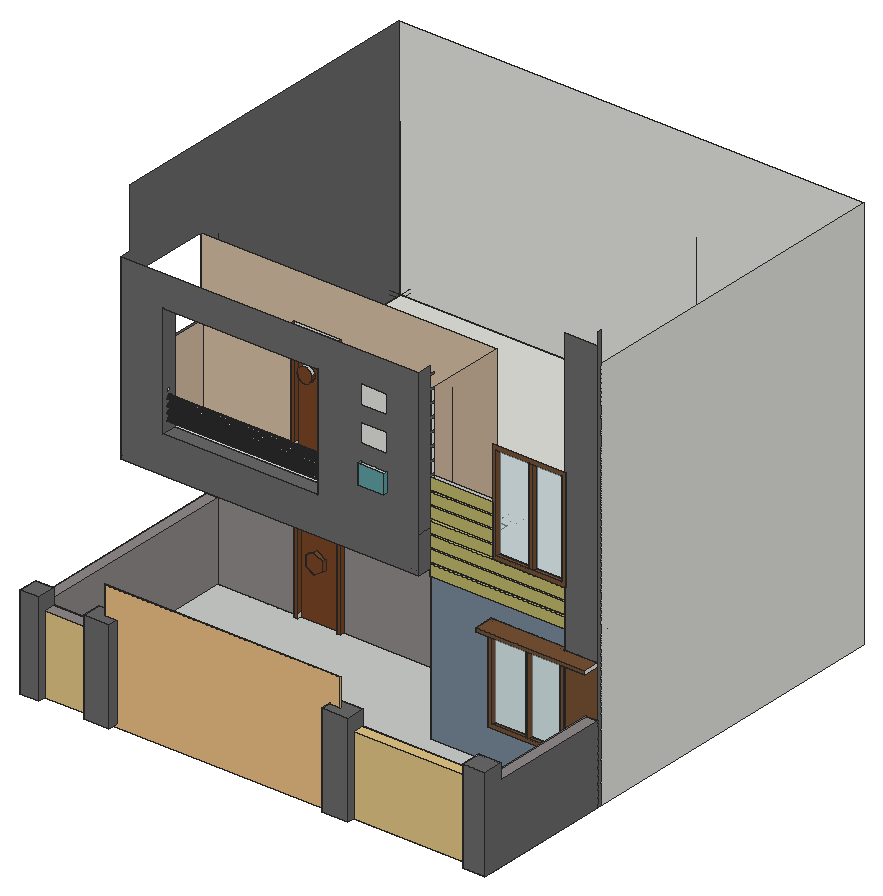
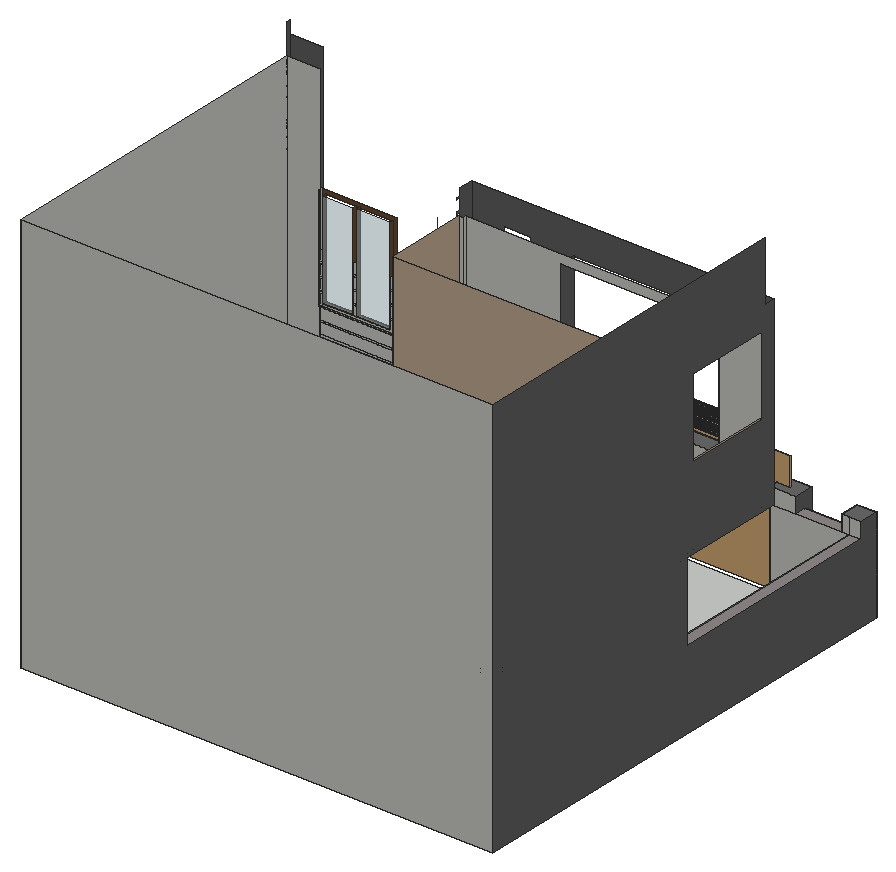
# SketchUp Ruby script. Lengths in inches.
U = 1.inch
M = Sketchup.active_model
def pt(a) = Geom::Point3d.new(a.map { |v| v * U })
def face(e, loops, mat)
  f = e.add_face(loops[0].map { |a| pt(a) })
  loops[1..].each { |l| e.add_face(l.map { |a| pt(a) }).erase! }
  f.material = f.back_material = mat if mat
  f
end
# faces: each face lists its corners as indices into pts; further lists are holes
def faces(e, pts, list, mat = nil) = list.each { |f| face(e, (f[0].is_a?(Array) ? f : [f]).map { |l| l.map { |i| pts[i] } }, mat) }
# xy, xz, yz: faces in a plane at the given z, y or x. An outline is a flat list of corners, or four numbers for a rectangle; further outlines are holes
def ring(l) = l.size == 4 ? [[l[0], l[1]], [l[2], l[1]], [l[2], l[3]], [l[0], l[3]]] : l.each_slice(2).to_a
def flat(e, list, mat, &to3) = list.each { |f| face(e, (f[0].is_a?(Array) ? f : [f]).map { |l| ring(l).map { |u, v| to3.(u, v) } }, mat) }
def xy(e, z, list, mat = nil) = flat(e, list, mat) { |x, y| [x, y, z] }
def xz(e, y, list, mat = nil) = flat(e, list, mat) { |x, z| [x, y, z] }
def yz(e, x, list, mat = nil) = flat(e, list, mat) { |y, z| [x, y, z] }
def lines(e, pts, list) = list.each { |a, b| e.add_line(pt(pts[a]), pt(pts[b])) }
# prism: a flat outline (further loops are holes) pulled along v
def prism(e, loops, v, mat = nil)
  f = face(e, loops, mat); d = Geom::Vector3d.new(v.map { |x| x * U })
  f.pushpull(f.normal.samedirection?(d) ? d.length : -d.length)
end
def box(e, o, s, mat = nil) = prism(e, [[o, [o[0] + s[0], o[1], o[2]], [o[0] + s[0], o[1] + s[1], o[2]], [o[0], o[1] + s[1], o[2]]]], [0, 0, s[2]], mat)
def at(x, y, z, deg = 0) = Geom::Transformation.translation(pt([x, y, z])) * Geom::Transformation.rotation(ORIGIN, Z_AXIS, deg.degrees)
def axes(o, x, y, z) = Geom::Transformation.new([*x, 0, *y, 0, *z, 0, *pt(o).to_a, 1])
def part(name) = M.definitions.add(name)
# library, detail: a bought-in or finely detailed component or shape, given as its bounding box
def library(name, o, s) = part(name).tap { |d| box(d.entities, o, s) }
def detail(e, o, s) = box(e.add_group.entities, o, s)
def put(e, d, t, mat = nil) = e.add_instance(d, t).tap { |i| i.material = mat if mat }
def group(e, t, mat = nil) = e.add_group.tap { |g| g.transformation = t; g.material = mat if mat }.entities
root = M.entities
M.materials.add("[0057_DarkKhaki]").color = [189, 183, 107]
M.materials.add("[0081_CadetBlue]").color = [95, 158, 160]
M.materials.add("[0110_LightSlateGray]").color = [119, 136, 153]
M.materials.add("[0134_DimGray]").color = [105, 105, 105]
M.materials.add("[Basic Tile]").color = [203, 206, 202]
M.materials.add("[Concrete Aggregate Smoke]").color = [154, 150, 148]
M.materials.add("[Formica Laminate Light]").color = [213, 189, 164]
M.materials.add("[Marble Carrara Gold Floor Tile]").color = [225, 223, 217]
M.materials.add("[Sandstone]").color = [118, 81, 52]
M.materials.add("[Stone Brushed Khaki]").color = [226, 197, 133]
M.materials.add("[Stone Marble]").color = [143, 138, 136]
M.materials.add("[Translucent Glass Safety]").color = [204, 235, 244]
M.materials["[Translucent Glass Safety]"].alpha = 0.5
M.materials.add("[Wood Veneer 01]").color = [120, 70, 37]
c1 = library("gate",[-17.08,19.83,-10.33],[162.44,1,145.04])
xy(root,0,[[0,0,14.57,6],[49.39,0,69.17,6],[233.33,0,233.33,15,351,15,351,108.71,360,108.71,360,6,253.41,6,253.41,0],[342.7,0,344.8125,6],[344.8125,0,360,6],
  [0,6,0,180.5,9,180.5,9,15,69.17,15,69.17,6],[334.9375,108.71,351,111.71],[351,108.71,360,111.71],[[228.875,111.71,228.875,180.5,0,180.5,0,366,360,366,360,111.71],[9,186.5,228.875,357],[234.875,117.71,351,357]],[234.875,117.71,351,357],
  [70.04,177.5,73.04,180.5],[103.04,177.5,106.04,180.5],[9,186.5,228.875,357]])
xy(root,0,[[9,15,351,15,351,108.71,334.9375,108.71,334.9375,111.71,228.875,111.71,228.875,180.5,106.04,180.5,106.04,177.5,103.04,177.5,103.04,180.5,73.04,180.5,73.04,177.5,70.04,177.5,70.04,180.5,9,180.5]],"[Basic Tile]")
xy(root,25.92,[[275.3,108.71,333.8,111.71]],"[Sandstone]")
xy(root,28.92,[[304.55,108.71,306.3125,111.71]])
xy(root,28.92,[[278.3,108.71,304.55,111.71],[306.3125,108.71,330.8,111.71]],"[Sandstone]")
xy(root,60,[[253.41,6,342.7,15]],"[Stone Brushed Khaki]")
xy(root,60,[[14.57,6,49.39,15],[0,15,9,180.5],[351,15,360,108.71]],"[Stone Marble]")
xy(root,72,[[0,0,14.57,15],[49.39,0,69.17,15],[233.33,0,253.41,15],[342.7,0,360,15]],"[0134_DimGray]")
xy(root,81,[[73.04,177.5,103.04,180.5]],"[Wood Veneer 01]")
xy(root,84,[[70.04,177.5,106.04,180.5]],"[Wood Veneer 01]")
xy(root,97.24,[[304.55,108.71,306.3125,111.71]])
xy(root,97.24,[[275.3,96.71,275.3,108.71,278.3,108.71,278.3,111.71,304.55,111.71,304.55,108.71,306.3125,108.71,306.3125,111.71,330.8,111.71,330.8,108.71,360,108.71,360,96.71]],"[Sandstone]")
xy(root,100.24,[[275.3,96.71,360,96.71,360,108.71,333.8,108.71,333.8,111.71,275.3,111.71]],"[Sandstone]")
xy(root,114.9375,[[230.5,111.71,334.9375,114.71]])
xy(root,114.9375,[[230.5,108.71,334.9375,111.71]],"[0057_DarkKhaki]")
xy(root,120,[[234.875,117.71,351,165.625],[228.875,165.625,234.875,180.4375],[234.875,165.625,234.875,180.4375,240,180.4375,240,357,351,357,351,165.625],[228.875,180.4375,234.875,180.5],[234.875,180.4375,240,186.5],
  [9,180.5,228.875,186.5],[228.875,180.5,234.875,186.5],[9,186.5,228.875,357],[228.875,186.5,234.875,357],[234.875,186.5,240,357]])
xy(root,120,[[0,97.375,0,180.5,228.875,180.5,228.875,111.71,230.5,111.71,230.5,97.375]],"[0134_DimGray]")
xy(root,123,[[237.875,120.71,237.875,174.625,9,174.625,9,357,351,357,351,120.71],[72.42,171.625,75.42,174.625],[75.42,171.625,105.42,174.625],[105.42,171.625,108.42,174.625],[108.42,171.625,228.875,174.625]])
xy(root,123.125,[[225.1875,109.375,228.875,111.71]])
xy(root,123.125,[[1.6875,109.375,225.1875,109.375,225.1875,111.71,228.875,111.71,228.875,171.625,72.42,171.625,72.42,174.625,1.6875,174.625]],"[Marble Carrara Gold Floor Tile]")
xy(root,123.41,[[230.5,111.71,334.9375,114.71]])
xy(root,123.41,[[230.5,108.71,334.9375,111.71]],"[0057_DarkKhaki]")
xy(root,124.9375,[[230.5,108.71,334.9375,111.71]],"[0057_DarkKhaki]")
xy(root,133.41,[[230.5,108.71,334.9375,111.71]],"[0057_DarkKhaki]")
xy(root,134.9375,[[230.5,108.71,334.9375,111.71]],"[0057_DarkKhaki]")
xy(root,143.41,[[230.5,108.71,334.9375,111.71]],"[0057_DarkKhaki]")
xy(root,143.82,[[278.53,108.71,334.9375,111.71],[334.9375,108.71,335.6,111.71]])
xy(root,144.9375,[[230.5,108.71,278.53,111.71]],"[0057_DarkKhaki]")
xy(root,146.82,[[307.0625,108.71,310.13,111.71]])
xy(root,146.82,[[281.53,108.71,307.0625,111.71],[310.13,108.71,332.6,111.71]],"[Sandstone]")
xy(root,148.61,[[32.625,97.375,152.93,109.375]],"[0134_DimGray]")
xy(root,153.41,[[230.5,108.71,278.53,111.71]],"[0057_DarkKhaki]")
xy(root,154.9375,[[230.5,108.71,278.53,111.71]],"[0057_DarkKhaki]")
xy(root,163.41,[[230.5,108.71,278.53,111.71]],"[0057_DarkKhaki]")
xy(root,164.9375,[[230.5,108.71,278.53,111.71]],"[0057_DarkKhaki]")
xy(root,168.75,[[185.74,94.375,206.18,97.375]],"[0081_CadetBlue]")
xy(root,173.41,[[230.5,108.71,278.53,111.71]],"[0057_DarkKhaki]")
xy(root,174.9375,[[230.5,108.71,278.53,111.71]],"[0057_DarkKhaki]")
xz(root,0,[[0,0,14.57,72],[49.39,0,69.17,72],[233.33,0,253.41,72],[342.7,0,360,72]],"[0134_DimGray]")
xz(root,6,[[14.57,0,49.39,60],[253.41,0,342.7,60]],"[Stone Brushed Khaki]")
xz(root,15,[[9,0,69.17,60],[233.33,0,233.33,72,253.41,72,253.41,60,351,60,351,0],[0,60,9,72],[9,60,14.57,72],[49.39,60,69.17,72],
  [342.7,60,344.8125,72],[344.8125,60,351,72],[351,60,360,72]])
xz(root,94.375,[[185.74,168.75,206.18,183.75]],"[0081_CadetBlue]")
xz(root,96.71,[[275.3,97.24,360,100.24]],"[Sandstone]")
xz(root,97.375,[[185.74,168.75,206.18,183.75]])
xz(root,97.375,[[[0,120,230.5,260.3125],[32.625,148.61,152.93,236.11],[185.74,222.6875,206.18,237.6875],[185.74,196.125,206.18,211.125],[185.74,168.75,206.18,183.75]]],"[0134_DimGray]")
xz(root,108.71,[[351,0,360,60],[333.8,97.24,334.9375,100.24],[334.9375,97.24,360,100.24]])
xz(root,108.71,[[230.5,114.9375,334.9375,123.41],[230.5,124.9375,334.9375,133.41],[230.5,134.9375,334.9375,143.41],[230.5,144.9375,278.53,153.41],[230.5,154.9375,278.53,163.41],
  [230.5,164.9375,278.53,173.41],[230.5,174.9375,278.53,183.41]],"[0057_DarkKhaki]")
xz(root,108.71,[[334.9375,100.24,360,100.24,360,320.08,334.9375,320.08,334.9375,223.14,335.6,223.14,335.6,143.82,334.9375,143.82]],"[0134_DimGray]")
xz(root,108.71,[[334.9375,0,351,0,351,60,360,60,360,97.24,334.9375,97.24],[275.3,25.92,333.8,25.92,333.8,97.24,330.8,97.24,330.8,28.92,278.3,28.92,278.3,97.24,275.3,97.24],[304.55,28.92,306.3125,97.24],[[278.53,143.82,335.6,223.14],[281.53,146.82,332.6,220.14]],[307.0625,146.82,310.13,220.14]],"[Sandstone]")
xz(root,109.375,[[1.6875,123.125,1.6875,183.125,0,183.125,0,243,152.93,243,152.93,236.11,32.625,236.11,32.625,148.61,152.93,148.61,152.93,243,225.1875,243,225.1875,123.125]])
xz(root,111.71,[[334.9375,0,334.9375,143.82,335.6,143.82,335.6,223.14,334.9375,223.14,334.9375,306,360,306,360,0],[[275.3,25.92,333.8,100.24],[278.3,28.92,330.8,97.24]],[304.55,28.92,306.3125,97.24],[230.5,114.9375,334.9375,123.41],[228.875,120,230.5,120.5625],
  [228.875,120.5625,230.5,243],[225.1875,123.125,228.875,243],[230.5,123.41,334.9375,124.9375],[230.5,124.9375,334.9375,133.41],[230.5,133.41,334.9375,134.9375],
  [230.5,134.9375,334.9375,143.41],[230.5,143.41,334.9375,143.41,334.9375,143.82,278.53,143.82,278.53,144.9375,230.5,144.9375],[278.53,143.82,334.9375,144.9375],[334.9375,143.82,335.6,223.14],[230.5,144.9375,278.53,153.41],
  [278.53,144.9375,334.9375,144.9375,334.9375,153.41,332.6,153.41,332.6,146.82,281.53,146.82,281.53,153.41,278.53,153.41],[307.0625,146.82,310.13,153.41],[230.5,153.41,278.53,154.9375],[278.53,153.41,281.53,154.9375],[307.0625,153.41,310.13,154.9375],
  [332.6,153.41,334.9375,154.9375],[230.5,154.9375,278.53,163.41],[278.53,154.9375,281.53,163.41],[307.0625,154.9375,310.13,163.41],[332.6,154.9375,334.9375,163.41],
  [230.5,163.41,278.53,164.9375],[278.53,163.41,281.53,164.9375],[307.0625,163.41,310.13,164.9375],[332.6,163.41,334.9375,164.9375],[230.5,164.9375,278.53,173.41],
  [278.53,164.9375,281.53,173.41],[307.0625,164.9375,310.13,173.41],[332.6,164.9375,334.9375,173.41],[230.5,173.41,278.53,174.9375],[278.53,173.41,281.53,174.9375],
  [307.0625,173.41,310.13,174.9375],[332.6,173.41,334.9375,174.9375],[230.5,174.9375,278.53,183.41],[278.53,174.9375,281.53,183.41],[307.0625,174.9375,310.13,183.41],
  [332.6,174.9375,334.9375,183.41]])
xz(root,111.71,[[[228.875,0,334.9375,0,334.9375,114.9375,230.5,114.9375,230.5,120,228.875,120],[275.3,25.92,333.8,100.24]]],"[0110_LightSlateGray]")
xz(root,111.71,[[278.3,28.92,304.55,97.24],[306.3125,28.92,330.8,97.24],[281.53,146.82,307.0625,220.14],[310.13,146.82,332.6,220.14]],"[Translucent Glass Safety]")
xz(root,114.71,[[230.5,114.9375,334.9375,123.41]])
xz(root,117.71,[[234.875,0,351,120]])
xz(root,171.625,[[72.42,123,75.42,123.125],[75.42,123,105.42,123.125],[105.42,123,108.42,123.125],[108.42,123,228.875,123.125]])
xz(root,171.625,[[72.42,123.125,75.42,123.125,75.42,204,105.42,204,105.42,123.125,108.42,123.125,108.42,207,72.42,207],[83.07,168.6875,84.55,168.91,85.93,169.51,87.1,170.44,88,171.65,88.55,173.04,88.72,174.53,88.5,176.02,87.9,177.39,86.97,178.57,85.76,179.46,84.37,180.02,82.875,180.1875,81.39,179.97,80.01,179.37,78.84,178.4375,77.94,177.23,77.39,175.83,77.22,174.34,77.44,172.86,78.04,171.48,78.97,170.31,80.18,169.41,81.57,168.86]],"[Wood Veneer 01]")
xz(root,174.625,[[72.42,123,72.42,207,108.42,207,108.42,123,105.42,123,105.42,204,75.42,204,75.42,123],[83.07,168.6875,81.57,168.86,80.18,169.41,78.97,170.31,78.04,171.48,77.44,172.86,77.22,174.34,77.39,175.83,77.94,177.23,78.84,178.4375,80.01,179.37,81.39,179.97,82.875,180.1875,84.37,180.02,85.76,179.46,86.97,178.57,87.9,177.39,88.5,176.02,88.72,174.53,88.55,173.04,88,171.65,87.1,170.44,85.93,169.51,84.55,168.91]])
xz(root,174.625,[[108.42,123,228.875,123,228.875,243,0,243,0,183.125,1.6875,183.125,1.6875,123.125,72.42,123.125,72.42,207,108.42,207]],"[Formica Laminate Light]")
xz(root,174.625,[[[75.42,123,105.42,204],[83.07,168.6875,81.57,168.86,80.18,169.41,78.97,170.31,78.04,171.48,77.44,172.86,77.22,174.34,77.39,175.83,77.94,177.23,78.84,178.4375,80.01,179.37,81.39,179.97,82.875,180.1875,84.37,180.02,85.76,179.46,86.97,178.57,87.9,177.39,88.5,176.02,88.72,174.53,88.55,173.04,88,171.65,87.1,170.44,85.93,169.51,84.55,168.91]]],"[Wood Veneer 01]")
xz(root,177.5,[[70.04,0,73.04,0,73.04,81,103.04,81,103.04,0,106.04,0,106.04,84,70.04,84],[85.58,34.92,92.02,38.64,92.02,46.07,85.58,49.79,79.14,46.07,79.14,38.64]],"[Wood Veneer 01]")
xz(root,180.5,[[70.04,0,70.04,84,106.04,84,106.04,0,103.04,0,103.04,81,73.04,81,73.04,0]])
xz(root,180.5,[[9,0,70.04,0,70.04,84,106.04,84,106.04,0,228.875,0,228.875,120,0,120,0,60,9,60]],"[Stone Marble]")
xz(root,180.5,[[[73.04,0,103.04,81],[85.58,34.92,79.14,38.64,79.14,46.07,85.58,49.79,92.02,46.07,92.02,38.64]]],"[Wood Veneer 01]")
xz(root,186.5,[[9,0,228.875,120]])
xz(root,357,[[9,0,228.875,120],[234.875,0,351,120],[9,120,228.875,123],[228.875,120,237.3125,123],[237.3125,120,240,123]])
xz(root,366,[[0,0,360,306]])
yz(root,0,[[[0,0,0,72,15,72,15,60,180.5,60,180.5,120,97.375,120,97.375,260.3125,106.375,260.3125,106.375,306,366,306,366,0],[109.375,183.125,174.625,243]]],"[0134_DimGray]")
yz(root,1.6875,[[109.375,123.125,174.625,183.125]],"[Formica Laminate Light]")
yz(root,9,[[186.5,0,357,120],[180.5,120,357,123]])
yz(root,9,[[15,0,180.5,60]],"[Stone Marble]")
yz(root,14.57,[[0,0,6,0,6,60,15,60,15,72,0,72]],"[0134_DimGray]")
yz(root,32.625,[[[97.375,148.61,109.375,236.11],[102.77,175.55,102.35,175.61,101.96,175.77,101.62,176.03,101.36,176.37,101.2,176.76,101.15,177.18,101.2,177.6,101.36,177.99,101.62,178.33,101.96,178.59,102.35,178.75,102.77,178.8,103.19,178.75,103.58,178.59,103.92,178.33,104.18,177.99,104.34,177.6,104.4,177.18,104.34,176.76,104.18,176.37,103.92,176.03,103.58,175.77,103.19,175.61],[102.77,170.55,102.35,170.61,101.96,170.77,101.62,171.03,101.36,171.37,101.2,171.76,101.15,172.18,101.2,172.6,101.36,172.99,101.62,173.33,101.96,173.59,102.35,173.75,102.77,173.8,103.19,173.75,103.58,173.59,103.92,173.33,104.18,172.99,104.34,172.6,104.4,172.18,104.34,171.76,104.18,171.37,103.92,171.03,103.58,170.77,103.19,170.61],[102.77,165.55,102.35,165.61,101.96,165.77,101.62,166.03,101.36,166.37,101.2,166.76,101.15,167.18,101.2,167.6,101.36,167.99,101.62,168.33,101.96,168.59,102.35,168.75,102.77,168.8,103.19,168.75,103.58,168.59,103.92,168.33,104.18,167.99,104.34,167.6,104.4,167.18,104.34,166.76,104.18,166.37,103.92,166.03,103.58,165.77,103.19,165.61],[102.77,160.55,102.35,160.61,101.96,160.77,101.62,161.03,101.36,161.37,101.2,161.76,101.15,162.18,101.2,162.6,101.36,162.99,101.62,163.33,101.96,163.59,102.35,163.75,102.77,163.8,103.19,163.75,103.58,163.59,103.92,163.33,104.18,162.99,104.34,162.6,104.4,162.18,104.34,161.76,104.18,161.37,103.92,161.03,103.58,160.77,103.19,160.61],[102.77,155.55,102.35,155.61,101.96,155.77,101.62,156.03,101.36,156.37,101.2,156.76,101.15,157.18,101.2,157.6,101.36,157.99,101.62,158.33,101.96,158.59,102.35,158.75,102.77,158.8,103.19,158.75,103.58,158.59,103.92,158.33,104.18,157.99,104.34,157.6,104.4,157.18,104.34,156.76,104.18,156.37,103.92,156.03,103.58,155.77,103.19,155.61]]],"[0134_DimGray]")
yz(root,49.39,[[0,0,0,72,15,72,15,60,6,60,6,0]],"[0134_DimGray]")
yz(root,69.17,[[0,0,15,72]],"[0134_DimGray]")
yz(root,70.04,[[177.5,0,180.5,84]],"[Wood Veneer 01]")
yz(root,72.42,[[171.625,123,174.625,123.125]])
yz(root,72.42,[[171.625,123.125,174.625,207]],"[Wood Veneer 01]")
yz(root,73.04,[[177.5,0,180.5,3]])
yz(root,73.04,[[177.5,3,180.5,81]],"[Wood Veneer 01]")
yz(root,75.42,[[171.625,123,174.625,126]])
yz(root,75.42,[[171.625,126,174.625,204]],"[Wood Veneer 01]")
yz(root,79.14,[[177.5,38.64,180.5,46.07]],"[Wood Veneer 01]")
yz(root,92.02,[[177.5,38.64,180.5,46.07]],"[Wood Veneer 01]")
yz(root,103.04,[[177.5,0,180.5,3]])
yz(root,103.04,[[177.5,3,180.5,81]],"[Wood Veneer 01]")
yz(root,105.42,[[171.625,123,174.625,126]])
yz(root,105.42,[[171.625,126,174.625,204]],"[Wood Veneer 01]")
yz(root,106.04,[[177.5,0,180.5,84]],"[Wood Veneer 01]")
yz(root,108.42,[[171.625,123,174.625,207]],"[Wood Veneer 01]")
yz(root,152.4375,[[102.77,160.55,103.19,160.61,103.58,160.77,103.92,161.03,104.18,161.37,104.34,161.76,104.4,162.18,104.34,162.6,104.18,162.99,103.92,163.33,103.58,163.59,103.19,163.75,102.77,163.8,102.35,163.75,101.96,163.59,101.62,163.33,101.36,162.99,101.2,162.6,101.15,162.18,101.2,161.76,101.36,161.37,101.62,161.03,101.96,160.77,102.35,160.61]])
yz(root,152.5625,[[102.77,170.55,103.19,170.61,103.58,170.77,103.92,171.03,104.18,171.37,104.34,171.76,104.4,172.18,104.34,172.6,104.18,172.99,103.92,173.33,103.58,173.59,103.19,173.75,102.77,173.8,102.35,173.75,101.96,173.59,101.62,173.33,101.36,172.99,101.2,172.6,101.15,172.18,101.2,171.76,101.36,171.37,101.62,171.03,101.96,170.77,102.35,170.61]])
yz(root,152.93,[[[97.375,148.61,109.375,236.11],[102.77,165.55,103.19,165.61,103.58,165.77,103.92,166.03,104.18,166.37,104.34,166.76,104.4,167.18,104.34,167.6,104.18,167.99,103.92,168.33,103.58,168.59,103.19,168.75,102.77,168.8,102.35,168.75,101.96,168.59,101.62,168.33,101.36,167.99,101.2,167.6,101.15,167.18,101.2,166.76,101.36,166.37,101.62,166.03,101.96,165.77,102.35,165.61],[102.77,155.55,103.19,155.61,103.58,155.77,103.92,156.03,104.18,156.37,104.34,156.76,104.4,157.18,104.34,157.6,104.18,157.99,103.92,158.33,103.58,158.59,103.19,158.75,102.77,158.8,102.35,158.75,101.96,158.59,101.62,158.33,101.36,157.99,101.2,157.6,101.15,157.18,101.2,156.76,101.36,156.37,101.62,156.03,101.96,155.77,102.35,155.61]]],"[0134_DimGray]")
yz(root,185.74,[[94.375,168.75,97.375,183.75]],"[0081_CadetBlue]")
yz(root,206.18,[[94.375,168.75,97.375,183.75]],"[0081_CadetBlue]")
yz(root,225.1875,[[109.375,123.125,111.71,243]])
yz(root,228.875,[[186.5,0,357,120],[111.71,120,171.625,123.125],[180.4375,120,180.5,123]])
yz(root,228.875,[[111.71,0,180.5,120]],"[0110_LightSlateGray]")
yz(root,228.875,[[171.625,123,171.625,123.125,111.71,123.125,111.71,243,174.625,243,174.625,123]],"[Formica Laminate Light]")
yz(root,230.5,[[111.71,114.9375,114.71,120],[108.71,120,109.375,120.5625],[109.375,120,111.71,120.5625],[111.71,120,114.71,120.5625],[108.71,120.5625,109.375,123.125],
  [109.375,120.5625,111.71,123.41],[111.71,120.5625,114.71,123.41],[108.71,123.125,109.375,123.41],[108.71,124.9375,109.375,133.41],[109.375,124.9375,111.71,133.41],
  [109.375,133.41,111.71,134.9375],[108.71,134.9375,109.375,143.41],[109.375,134.9375,111.71,143.41],[109.375,143.41,111.71,144.9375],[108.71,144.9375,109.375,148.61],
  [109.375,144.9375,111.71,144.9375,111.71,153.41,108.71,153.41,108.71,148.61,109.375,148.61],[108.71,154.9375,111.71,163.41],[108.71,164.9375,111.71,173.41],[108.71,174.9375,111.71,183.41]])
yz(root,230.5,[[108.71,114.9375,111.71,120]],"[0057_DarkKhaki]")
yz(root,230.5,[[97.375,120,108.71,120,108.71,123.41,111.71,123.41,111.71,124.9375,108.71,124.9375,108.71,133.41,109.375,133.41,109.375,134.9375,108.71,134.9375,108.71,143.41,109.375,143.41,109.375,144.9375,108.71,144.9375,108.71,148.61,97.375,148.61],[97.375,148.61,108.71,148.61,108.71,153.41,111.71,153.41,111.71,154.9375,108.71,154.9375,108.71,163.41,111.71,163.41,111.71,164.9375,108.71,164.9375,108.71,173.41,111.71,173.41,111.71,174.9375,108.71,174.9375,108.71,183.41,111.71,183.41,111.71,184.9375,108.71,184.9375,108.71,193.41,111.71,193.41,111.71,194.9375,108.71,194.9375,108.71,203.41,111.71,203.41,111.71,204.9375,108.71,204.9375,108.71,213.41,111.71,213.41,111.71,214.9375,108.71,214.9375,108.71,223.41,111.71,223.41,111.71,224.9375,108.71,224.9375,108.71,233.41,111.71,233.41,111.71,234.9375,108.71,234.9375,108.71,243.41,111.71,243.41,111.71,244.9375,108.71,244.9375,108.71,253.41,111.71,253.41,111.71,254.9375,108.71,254.9375,108.71,260.3125,97.375,260.3125]],"[0134_DimGray]")
yz(root,233.33,[[0,0,15,72]],"[0134_DimGray]")
yz(root,234.875,[[117.71,0,357,120]])
yz(root,253.41,[[0,0,6,0,6,60,15,60,15,72,0,72]],"[0134_DimGray]")
yz(root,275.3,[[108.71,25.92,111.71,100.24],[96.71,97.24,108.71,100.24]],"[Sandstone]")
yz(root,278.3,[[108.71,28.92,111.71,97.24]],"[Sandstone]")
yz(root,278.53,[[108.71,143.82,111.71,144.9375],[108.71,144.9375,111.71,153.41],[108.71,153.41,111.71,154.9375],[108.71,154.9375,111.71,163.41],[108.71,163.41,111.71,164.9375],
  [108.71,164.9375,111.71,173.41],[108.71,173.41,111.71,174.9375],[108.71,174.9375,111.71,183.41]])
yz(root,281.53,[[108.71,146.82,111.71,220.14]],"[Sandstone]")
yz(root,304.55,[[108.71,28.92,111.71,97.24]],"[Sandstone]")
yz(root,306.3125,[[108.71,28.92,111.71,97.24]],"[Sandstone]")
yz(root,307.0625,[[108.71,146.82,111.71,220.14]],"[Sandstone]")
yz(root,310.13,[[108.71,146.82,111.71,220.14]],"[Sandstone]")
yz(root,330.8,[[108.71,28.92,111.71,97.24]],"[Sandstone]")
yz(root,332.6,[[108.71,146.82,111.71,220.14]],"[Sandstone]")
yz(root,333.8,[[108.71,25.92,111.71,100.24]],"[Sandstone]")
yz(root,334.9375,[[108.71,0,111.71,114.9375],[108.71,114.9375,111.71,123.41],[111.71,114.9375,114.71,123.41],[108.71,123.41,111.71,124.9375],[108.71,124.9375,111.71,133.41],
  [108.71,133.41,111.71,134.9375],[108.71,134.9375,111.71,143.41],[108.71,143.41,111.71,143.82]])
yz(root,335.6,[[108.71,143.82,111.71,223.14]])
yz(root,342.7,[[0,0,0,72,15,72,15,60,6,60,6,0]])
yz(root,351,[[117.71,0,357,120]])
yz(root,351,[[15,0,108.71,60]],"[Stone Marble]")
yz(root,360,[[111.71,0,366,306],[96.71,97.24,108.71,100.24]])
yz(root,360,[[0,0,108.71,0,108.71,60,15,60,15,72,0,72],[108.71,0,111.71,329.5]],"[0134_DimGray]")
p = [[79.14,180.5,38.64],[85.58,180.5,34.92],[85.58,177.5,34.92],[79.14,177.5,38.64],[92.02,180.5,38.64],[92.02,177.5,38.64],
  [85.58,180.5,49.79],[79.14,180.5,46.07],[79.14,177.5,46.07],[85.58,177.5,49.79],[92.02,180.5,46.07],[92.02,177.5,46.07],
  [32.625,101.96,155.77],[32.625,102.35,155.61],[152.93,102.35,155.61],[152.93,101.96,155.77],[32.625,102.77,155.55],[152.93,102.77,155.55],
  [32.625,103.19,155.61],[152.93,103.19,155.61],[32.625,103.58,155.77],[152.93,103.58,155.77],[32.625,101.62,156.03],[152.93,101.62,156.03],
  [32.625,103.92,156.03],[152.93,103.92,156.03],[32.625,101.36,156.37],[152.93,101.36,156.37],[32.625,104.18,156.37],[152.93,104.18,156.37],
  [32.625,101.2,156.76],[152.93,101.2,156.76],[32.625,104.34,156.76],[152.93,104.34,156.76],[32.625,101.15,157.18],[152.93,101.15,157.18],
  [32.625,104.4,157.18],[152.93,104.4,157.18],[32.625,101.2,157.6],[152.93,101.2,157.6],[32.625,104.34,157.6],[152.93,104.34,157.6],
  [32.625,101.36,157.99],[152.93,101.36,157.99],[32.625,104.18,157.99],[152.93,104.18,157.99],[32.625,101.62,158.33],[152.93,101.62,158.33],
  [32.625,103.92,158.33],[152.93,103.92,158.33],[32.625,101.96,158.59],[152.93,101.96,158.59],[32.625,103.58,158.59],[152.93,103.58,158.59],
  [32.625,102.35,158.75],[152.93,102.35,158.75],[32.625,103.19,158.75],[152.93,103.19,158.75],[32.625,102.77,158.8],[152.93,102.77,158.8],
  [32.625,101.96,160.77],[32.625,102.35,160.61],[152.4375,102.35,160.61],[152.4375,101.96,160.77],[32.625,102.77,160.55],[152.4375,102.77,160.55],
  [32.625,103.19,160.61],[152.4375,103.19,160.61],[32.625,103.58,160.77],[152.4375,103.58,160.77],[32.625,101.62,161.03],[152.4375,101.62,161.03],
  [32.625,103.92,161.03],[152.4375,103.92,161.03],[32.625,101.36,161.37],[152.4375,101.36,161.37],[32.625,104.18,161.37],[152.4375,104.18,161.37],
  [32.625,101.2,161.76],[152.4375,101.2,161.76],[32.625,104.34,161.76],[152.4375,104.34,161.76],[32.625,101.15,162.18],[152.4375,101.15,162.18],
  [32.625,104.4,162.18],[152.4375,104.4,162.18],[32.625,101.2,162.6],[152.4375,101.2,162.6],[32.625,104.34,162.6],[152.4375,104.34,162.6],
  [32.625,101.36,162.99],[152.4375,101.36,162.99],[32.625,104.18,162.99],[152.4375,104.18,162.99],[32.625,101.62,163.33],[152.4375,101.62,163.33],
  [32.625,103.92,163.33],[152.4375,103.92,163.33],[32.625,101.96,163.59],[152.4375,101.96,163.59],[32.625,103.58,163.59],[152.4375,103.58,163.59],
  [32.625,102.35,163.75],[152.4375,102.35,163.75],[32.625,103.19,163.75],[152.4375,103.19,163.75],[32.625,102.77,163.8],[152.4375,102.77,163.8],
  [32.625,101.96,165.77],[32.625,102.35,165.61],[152.93,102.35,165.61],[152.93,101.96,165.77],[32.625,102.77,165.55],[152.93,102.77,165.55],
  [32.625,103.19,165.61],[152.93,103.19,165.61],[32.625,103.58,165.77],[152.93,103.58,165.77],[32.625,101.62,166.03],[152.93,101.62,166.03],
  [32.625,103.92,166.03],[152.93,103.92,166.03],[32.625,101.36,166.37],[152.93,101.36,166.37],[32.625,104.18,166.37],[152.93,104.18,166.37],
  [32.625,101.2,166.76],[152.93,101.2,166.76],[32.625,104.34,166.76],[152.93,104.34,166.76],[32.625,101.15,167.18],[152.93,101.15,167.18],
  [32.625,104.4,167.18],[152.93,104.4,167.18],[32.625,101.2,167.6],[152.93,101.2,167.6],[32.625,104.34,167.6],[152.93,104.34,167.6],
  [32.625,101.36,167.99],[152.93,101.36,167.99],[32.625,104.18,167.99],[152.93,104.18,167.99],[32.625,101.62,168.33],[152.93,101.62,168.33],
  [32.625,103.92,168.33],[152.93,103.92,168.33],[32.625,101.96,168.59],[152.93,101.96,168.59],[32.625,103.58,168.59],[152.93,103.58,168.59],
  [32.625,102.35,168.75],[152.93,102.35,168.75],[32.625,103.19,168.75],[152.93,103.19,168.75],[32.625,102.77,168.8],[152.93,102.77,168.8],
  [81.57,174.625,168.86],[83.07,174.625,168.6875],[83.07,171.625,168.6875],[81.57,171.625,168.86],[84.55,174.625,168.91],[84.55,171.625,168.91],
  [80.18,174.625,169.41],[80.18,171.625,169.41],[85.93,174.625,169.51],[85.93,171.625,169.51],[78.97,174.625,170.31],[78.97,171.625,170.31],
  [87.1,174.625,170.44],[87.1,171.625,170.44],[78.04,174.625,171.48],[78.04,171.625,171.48],[88,174.625,171.65],[88,171.625,171.65],
  [32.625,101.96,170.77],[32.625,102.35,170.61],[152.5625,102.35,170.61],[152.5625,101.96,170.77],[32.625,102.77,170.55],[152.5625,102.77,170.55],
  [32.625,103.19,170.61],[152.5625,103.19,170.61],[32.625,103.58,170.77],[152.5625,103.58,170.77],[32.625,101.62,171.03],[152.5625,101.62,171.03],
  [32.625,103.92,171.03],[152.5625,103.92,171.03],[32.625,101.36,171.37],[152.5625,101.36,171.37],[32.625,104.18,171.37],[152.5625,104.18,171.37],
  [32.625,101.2,171.76],[152.5625,101.2,171.76],[32.625,104.34,171.76],[152.5625,104.34,171.76],[77.44,174.625,172.86],[77.44,171.625,172.86],
  [88.55,174.625,173.04],[88.55,171.625,173.04],[32.625,101.15,172.18],[152.5625,101.15,172.18],[32.625,104.4,172.18],[152.5625,104.4,172.18],
  [32.625,101.2,172.6],[152.5625,101.2,172.6],[32.625,104.34,172.6],[152.5625,104.34,172.6],[32.625,101.36,172.99],[152.5625,101.36,172.99],
  [32.625,104.18,172.99],[152.5625,104.18,172.99],[77.22,174.625,174.34],[77.22,171.625,174.34],[32.625,101.62,173.33],[152.5625,101.62,173.33],
  [32.625,103.92,173.33],[152.5625,103.92,173.33],[88.72,174.625,174.53],[88.72,171.625,174.53],[32.625,101.96,173.59],[152.5625,101.96,173.59],
  [32.625,103.58,173.59],[152.5625,103.58,173.59],[32.625,102.35,173.75],[152.5625,102.35,173.75],[32.625,103.19,173.75],[152.5625,103.19,173.75],
  [32.625,102.77,173.8],[152.5625,102.77,173.8],[77.39,174.625,175.83],[77.39,171.625,175.83],[88.5,174.625,176.02],[88.5,171.625,176.02],
  [330.1,111.71,120],[330.1,117.71,120],[228.875,186.5,120],[228.875,186.5,123],[9,357,120],[0,357,120],
  [9,186.5,120],[0,186.5,120],[234.875,180.5,120],[234.875,180.5,123],[234.875,165.625,120],[234.875,165.625,123],
  [234.875,117.71,120],[234.875,111.71,120],[351,117.71,120],[360,117.71,120],[240,186.5,120],[240,186.5,123],
  [9,366,120],[240,180.4375,120],[240,180.4375,123],[234.875,180.4375,123],[237.3125,357,123],[237.3125,357,243],
  [9,357,123],[9,357,243],[9,180.5,123],[9,180.5,243],[237.875,120.71,123],[237.875,120.71,243],
  [0,357,123],[9,366,123],[351,120.71,123],[351,111.71,123],[237.875,111.71,123],[228.875,120.71,123],
  [0,174.625,123],[0,174.625,123.125],[0,180.5,123],[0,109.375,123.125],[1.6875,109.375,123.125],[228.875,109.375,123.125],
  [230.5,109.375,123.125],[228.875,111.71,120.5625],[228.875,109.375,120.5625],[278.3,108.71,97.24],[278.3,108.71,100.24],[330.8,108.71,97.24],
  [330.8,108.71,100.24],[9,174.625,123],[1.6875,174.625,123.125],[1.6875,97.375,123.125],[225.1875,109.375,123.125],[225.1875,97.375,123.125],
  [228.875,97.375,123.125],[344.8125,6,0],[344.8125,15,60]]
faces(root,p,[[0,1,2,3],[1,4,5,2],[6,7,8,9],[10,6,9,11],[156,157,158,159],[157,160,161,158],[162,156,159,163],[160,164,165,161],
  [166,162,163,167],[164,168,169,165],[170,166,167,171],[168,172,173,169],[196,170,171,197],[172,198,199,173],[212,196,197,213],[198,218,219,199],
  [230,212,213,231],[218,232,233,219]],"[Wood Veneer 01]")
faces(root,p,[[12,13,14,15],[13,16,17,14],[16,18,19,17],[18,20,21,19],[22,12,15,23],[20,24,25,21],[26,22,23,27],[24,28,29,25],
  [30,26,27,31],[28,32,33,29],[34,30,31,35],[32,36,37,33],[38,34,35,39],[36,40,41,37],[42,38,39,43],[40,44,45,41],
  [46,42,43,47],[44,48,49,45],[50,46,47,51],[48,52,53,49],[54,50,51,55],[52,56,57,53],[58,54,55,59],[56,58,59,57],
  [60,61,62,63],[61,64,65,62],[64,66,67,65],[66,68,69,67],[70,60,63,71],[68,72,73,69],[74,70,71,75],[72,76,77,73],
  [78,74,75,79],[76,80,81,77],[82,78,79,83],[80,84,85,81],[86,82,83,87],[84,88,89,85],[90,86,87,91],[88,92,93,89],
  [94,90,91,95],[92,96,97,93],[98,94,95,99],[96,100,101,97],[102,98,99,103],[100,104,105,101],[106,102,103,107],[104,106,107,105],
  [108,109,110,111],[109,112,113,110],[112,114,115,113],[114,116,117,115],[118,108,111,119],[116,120,121,117],[122,118,119,123],[120,124,125,121],
  [126,122,123,127],[124,128,129,125],[130,126,127,131],[128,132,133,129],[134,130,131,135],[132,136,137,133],[138,134,135,139],[136,140,141,137],
  [142,138,139,143],[140,144,145,141],[146,142,143,147],[144,148,149,145],[150,146,147,151],[148,152,153,149],[154,150,151,155],[152,154,155,153],
  [174,175,176,177],[175,178,179,176],[178,180,181,179],[180,182,183,181],[184,174,177,185],[182,186,187,183],[188,184,185,189],[186,190,191,187],
  [192,188,189,193],[190,194,195,191],[200,192,193,201],[194,202,203,195],[204,200,201,205],[202,206,207,203],[208,204,205,209],[206,210,211,207],
  [214,208,209,215],[210,216,217,211],[220,214,215,221],[216,222,223,217],[224,220,221,225],[222,226,227,223],[228,224,225,229],[226,228,229,227]],"[Concrete Aggregate Smoke]")
lines(root,p,[[234,235],[236,237],[238,239],[240,241],[242,243],[244,245],[246,247],[248,249],[250,251],[238,252],[253,254],[243,255],
  [256,257],[258,259],[260,261],[262,263],[258,264],[258,265],[266,267],[262,268],[262,269],[270,271],[260,272],[273,274],
  [275,276],[277,278],[279,280],[281,282],[270,283],[271,284],[274,285],[286,287],[275,288],[289,290]])
put(root,c1,axes([78.51,-5.38,4.39],[1.122,0,0],[0,0.66,0],[0,0,0.66]))
